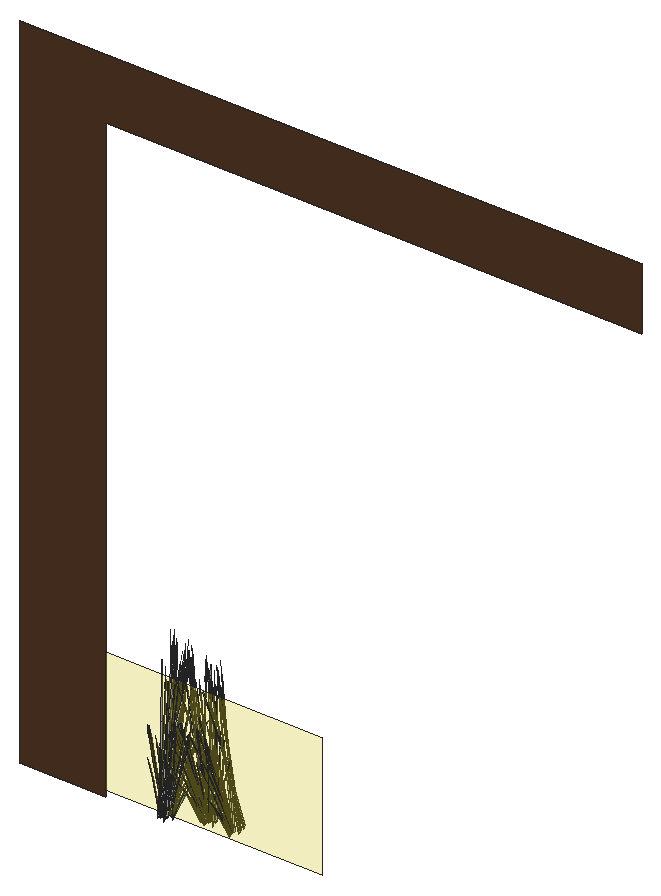
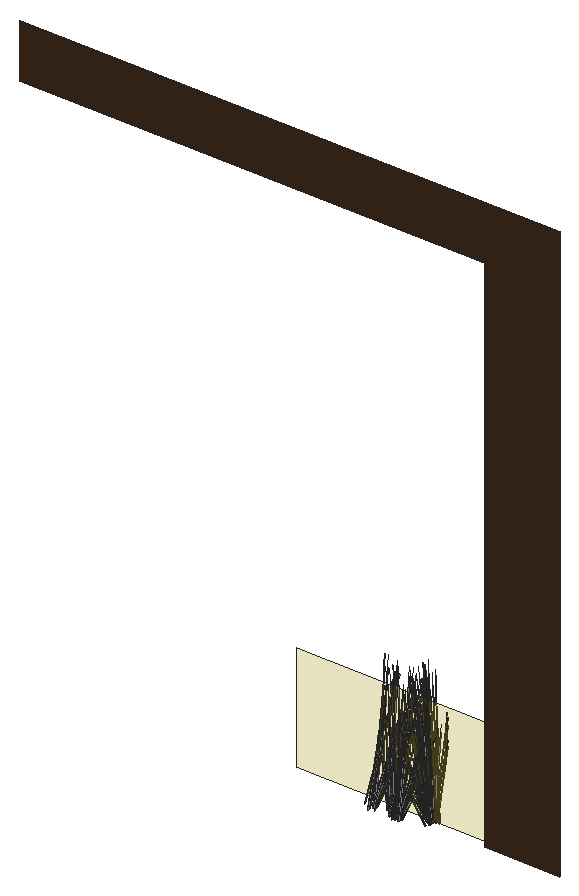
# SketchUp Ruby script. Lengths in inches.
U = 1.inch
M = Sketchup.active_model
def pt(a) = Geom::Point3d.new(a.map { |v| v * U })
def face(e, loops, mat)
  f = e.add_face(loops[0].map { |a| pt(a) })
  loops[1..].each { |l| e.add_face(l.map { |a| pt(a) }).erase! }
  f.material = f.back_material = mat if mat
  f
end
# faces: each face lists its corners as indices into pts; further lists are holes
def faces(e, pts, list, mat = nil) = list.each { |f| face(e, (f[0].is_a?(Array) ? f : [f]).map { |l| l.map { |i| pts[i] } }, mat) }
# xy, xz, yz: faces in a plane at the given z, y or x. An outline is a flat list of corners, or four numbers for a rectangle; further outlines are holes
def ring(l) = l.size == 4 ? [[l[0], l[1]], [l[2], l[1]], [l[2], l[3]], [l[0], l[3]]] : l.each_slice(2).to_a
def flat(e, list, mat, &to3) = list.each { |f| face(e, (f[0].is_a?(Array) ? f : [f]).map { |l| ring(l).map { |u, v| to3.(u, v) } }, mat) }
def xy(e, z, list, mat = nil) = flat(e, list, mat) { |x, y| [x, y, z] }
def xz(e, y, list, mat = nil) = flat(e, list, mat) { |x, z| [x, y, z] }
def yz(e, x, list, mat = nil) = flat(e, list, mat) { |y, z| [x, y, z] }
def lines(e, pts, list) = list.each { |a, b| e.add_line(pt(pts[a]), pt(pts[b])) }
# prism: a flat outline (further loops are holes) pulled along v
def prism(e, loops, v, mat = nil)
  f = face(e, loops, mat); d = Geom::Vector3d.new(v.map { |x| x * U })
  f.pushpull(f.normal.samedirection?(d) ? d.length : -d.length)
end
def box(e, o, s, mat = nil) = prism(e, [[o, [o[0] + s[0], o[1], o[2]], [o[0] + s[0], o[1] + s[1], o[2]], [o[0], o[1] + s[1], o[2]]]], [0, 0, s[2]], mat)
def at(x, y, z, deg = 0) = Geom::Transformation.translation(pt([x, y, z])) * Geom::Transformation.rotation(ORIGIN, Z_AXIS, deg.degrees)
def axes(o, x, y, z) = Geom::Transformation.new([*x, 0, *y, 0, *z, 0, *pt(o).to_a, 1])
def part(name) = M.definitions.add(name)
# library, detail: a bought-in or finely detailed component or shape, given as its bounding box
def library(name, o, s) = part(name).tap { |d| box(d.entities, o, s) }
def detail(e, o, s) = box(e.add_group.entities, o, s)
def put(e, d, t, mat = nil) = e.add_instance(d, t).tap { |i| i.material = mat if mat }
def group(e, t, mat = nil) = e.add_group.tap { |g| g.transformation = t; g.material = mat if mat }.entities
root = M.entities
M.materials.add("Glass_Basic_01").color = [255, 228, 0]
M.materials["Glass_Basic_01"].alpha = 0.25
M.materials.add("LightPink_Translucent").color = [144, 107, 117]
M.materials["LightPink_Translucent"].alpha = 0.75
M.materials.add("Wood_Veneer_15_1K").color = [81, 54, 35]
M.materials.add("[_0053_Ivory_]").color = [200, 200, 200]
c1 = part("blade")
p = [[2.15,0.21,22],[0,0.17,0],[0.09,0.45,0],[2.18,0.31,22],[2.29,0.31,22],[0.38,0.45,0],
  [2.48,0.24,33],[2.49,0.24,33],[2.48,0.22,33]]
faces(c1.entities,p,[[0,1,2,3],[4,5,2,3],[6,3,4,7],[8,0,3,6]])
c2 = part("seeds")
p = [[0.3,-0.1,1.38],[-0.01,-0.03,1.59],[-0.01,-0.03,0.03],[0.14,-0.07,-0.07],[0.29,-0.03,3],[0.15,0.01,3.11]]
faces(c2.entities,p,[[0,1,2,3],[1,0,4,5]],"LightPink_Translucent")
c3 = part("blade with seeds")
put(c3.entities,c1,at(0,0,0))
put(c3.entities,c2,axes([2.4,0.25,30.99],[1.5799,-0.05474,1.17369],[-0.12525,1.92788,0.29478],[-0.07173,-0.02425,1.56792]))
xz(root,98.15,[[410.51,129,494.51,177]],"Glass_Basic_01")
xz(root,98.15,[[377.51,127,410.51,127,410.51,360,617.51,360,617.51,384,377.51,384]],"Wood_Veneer_15_1K")
put(root,c3,axes([433.86,95.57,129.24],[-0.17264,0.12729,1.43002],[-0.51703,-0.22279,-0.30754],[0.09584,-0.27707,0.61141]),"[_0053_Ivory_]")
put(root,c3,axes([434.28,96.52,131.63],[0.0158,-0.58168,-0.71045],[0.66548,0.03907,0.08574],[0.07023,-0.24643,1.00501]),"[_0053_Ivory_]")
put(root,c3,axes([433.53,96.22,130.53],[-0.11309,0.21615,1.71376],[-0.47441,-0.44731,0.13857],[0.21402,-0.27879,0.73262]),"[_0053_Ivory_]")
put(root,c3,axes([434.14,96.32,131.33],[-0.43478,-0.42253,-0.51099],[0.45929,-0.37004,-0.3958],[0.06615,-0.21468,0.97773]),"[_0053_Ivory_]")
put(root,c3,axes([434.55,96.17,131.18],[0.41095,-0.33109,-0.35414],[0.38901,0.37805,0.4572],[0.05919,-0.19208,0.87481]),"[_0053_Ivory_]")
put(root,c3,axes([435.0625,95.97,128.15],[-0.0909,-0.04954,1.76342],[-0.2335,-0.55347,-0.26939],[0.15752,-0.1502,0.30037]),"[_0053_Ivory_]")
put(root,c3,axes([435.0625,97.53,131.63],[0.31725,-0.49618,-0.71045],[0.55593,0.35263,0.08574],[0.18942,-0.17977,1.00501]),"[_0053_Ivory_]")
put(root,c3,axes([435.05,97.3,131.33],[-0.15602,-0.5742,-0.51099],[0.59087,-0.10045,-0.3958],[0.16933,-0.15423,0.97773]),"[_0053_Ivory_]")
put(root,c3,axes([432.15,95.99,128.67],[0.56842,-0.31443,-0.49651],[0.33976,0.56381,0],[0.12946,-0.07161,1.57504]),"[_0053_Ivory_]")
put(root,c3,axes([435.52,97.07,129.24],[-0.21697,-0.01863,1.43002],[-0.22228,-0.49966,-0.30754],[0.26655,-0.14135,0.61141]),"[_0053_Ivory_]")
put(root,c3,axes([432.82,97.28,128.71],[0.40909,-0.47266,-0.62353],[0.50819,0.4286,-0.16365],[0.16393,-0.11791,1.37633]),"[_0053_Ivory_]")
put(root,c3,axes([435.77,96.15,129.42],[-0.2023,0.32011,1.1486],[-0.17388,-0.43009,0.84392],[0.16708,-0.10777,0.25299]),"[_0053_Ivory_]")
put(root,c3,axes([435.48,97.36,131.18],[0.52868,-0.08987,-0.35414],[0.1396,0.51376,0.4572],[0.1515,-0.13799,0.87481]),"[_0053_Ivory_]")
put(root,c3,axes([432.38,97.82,129.32],[-0.07077,-0.71755,-0.29095],[0.73712,-0.04339,-0.50002],[0.1298,-0.09558,1.59708]),"[_0053_Ivory_]")
put(root,c3,axes([432.28,96.23,128.68],[0.56663,0.1556,-0.30978],[-0.14267,0.54795,0.30978],[0.11423,-0.06319,1.38974]),"[_0053_Ivory_]")
put(root,c3,axes([457.25,100.86,130.53],[0.13883,0.2019,1.71376],[-0.64153,0.16998,0.13857],[-0.14499,-0.31697,0.73262]),"[_0053_Ivory_]")
put(root,c3,axes([457.07,100.32,129.24],[-0.03678,0.20572,1.43002],[-0.53767,0.17221,-0.30754],[-0.12568,-0.26589,0.61141]),"[_0053_Ivory_]")
put(root,c3,axes([435.32,98.57,131.33],[0.16454,-0.57202,-0.51099],[0.56413,0.19607,-0.3958],[0.22713,-0.05245,0.97773]),"[_0053_Ivory_]")
put(root,c3,axes([434.43,96.24,129.03],[0.37973,-0.63014,0],[0.6353,0.35142,-0.51607],[0.14469,0.08004,1.63711]),"[_0053_Ivory_]")
put(root,c3,axes([435.92,98.73,128.64],[-0.39118,0.07547,1.41583],[-0.06226,-0.6007,0.08104],[0.27398,-0.09092,0.80566]),"[_0053_Ivory_]")
put(root,c3,axes([436.63,98.2,128.91],[-0.37654,-0.40212,-0.06488],[0.4124,-0.36845,-0.29416],[0.11685,-0.02594,0.97024]),"[_0053_Ivory_]")
put(root,c3,axes([444.76,102.68,130.53],[0.13883,0.2019,1.71376],[-0.64153,0.16998,0.13857],[-0.14499,-0.31697,0.73262]),"[_0053_Ivory_]")
put(root,c3,axes([456.88,99.99,129.42],[0.31682,0.21887,1.1486],[-0.4614,0.13157,0.84392],[-0.09872,-0.16821,0.25299]),"[_0053_Ivory_]")
put(root,c3,axes([434.1,96.57,129.13],[-0.56842,-0.31443,0.49651],[0.33976,-0.56381,0],[0.12946,0.07161,1.57504]),"[_0053_Ivory_]")
put(root,c3,axes([457.65,101.15,131.63],[-0.51789,-0.30395,-0.71045],[0.36805,-0.53263,0.08574],[-0.18764,-0.18149,1.00501]),"[_0053_Ivory_]")
put(root,c3,axes([435.21,98.78,131.63],[0.53369,-0.27773,-0.71045],[0.29743,0.5717,0.08574],[0.25786,-0.06494,1.00501]),"[_0053_Ivory_]")
put(root,c3,axes([457.47,100.75,131.18],[-0.0938,-0.50652,-0.35414],[0.53623,-0.13375,0.4572],[-0.14403,-0.14515,0.87481]),"[_0053_Ivory_]")
put(root,c3,axes([447.26,102.38,129.24],[-0.17264,0.12729,1.43002],[-0.51703,-0.22279,-0.30754],[0.09584,-0.27707,0.61141]),"[_0053_Ivory_]")
put(root,c3,axes([446.47,102.83,131.63],[-0.28988,-0.51132,-0.71045],[0.59671,-0.28496,0.08574],[-0.06778,-0.24706,1.00501]),"[_0053_Ivory_]")
put(root,c3,axes([444.59,102.14,129.24],[-0.03678,0.20572,1.43002],[-0.53767,0.17221,-0.30754],[-0.12568,-0.26589,0.61141]),"[_0053_Ivory_]")
put(root,c3,axes([431.68,97.36,128.25],[-0.59782,0.25177,1.28929],[-0.19028,-0.72239,0.50096],[0.36709,0.01202,1.46642]),"[_0053_Ivory_]")
put(root,c3,axes([433.29,97.55,129.27],[0.11717,-0.56122,0.1448],[0.57245,0.09742,-0.41347],[0.10418,0.05763,1.26744]),"[_0053_Ivory_]")
put(root,c3,axes([445.97,101.69,128.15],[-0.10187,0.02266,1.76342],[-0.56336,-0.25503,-0.26939],[0.00945,-0.21273,0.30037]),"[_0053_Ivory_]")
put(root,c3,axes([456.63,100.65,128.15],[-0.05883,0.08284,1.76342],[-0.59454,0.17861,-0.26939],[-0.14363,-0.16248,0.30037]),"[_0053_Ivory_]")
put(root,c3,axes([436.35,98.34,128.15],[-0.03174,-0.09547,1.76342],[0.22015,-0.55846,-0.26939],[0.22208,-0.00803,0.30037]),"[_0053_Ivory_]")
put(root,c3,axes([456.32,101.49,130.53],[0.2256,0.10835,1.71376],[-0.46687,0.45453,0.13857],[-0.29098,-0.20505,0.73262]),"[_0053_Ivory_]")
put(root,c3,axes([447.68,103.33,131.63],[0.0158,-0.58168,-0.71045],[0.66548,0.03907,0.08574],[0.07023,-0.24643,1.00501]),"[_0053_Ivory_]")
put(root,c3,axes([433.04,97.7,129.37],[-0.36485,-0.52782,0.44739],[0.55265,-0.37168,-0.21531],[0.11807,0.06531,1.43643]),"[_0053_Ivory_]")
put(root,c3,axes([446.53,102.39,131.18],[0.1831,-0.48359,-0.35414],[0.53419,0.14105,0.4572],[-0.04898,-0.1947,0.87481]),"[_0053_Ivory_]")
put(root,c3,axes([446.93,103.03,130.53],[-0.11309,0.21615,1.71376],[-0.47441,-0.44731,0.13857],[0.21402,-0.27879,0.73262]),"[_0053_Ivory_]")
put(root,c3,axes([457.41,101.17,131.33],[-0.59932,0.14948,-0.51099],[-0.10484,-0.56611,-0.3958],[-0.16097,-0.16223,0.97773]),"[_0053_Ivory_]")
put(root,c3,axes([433.23,97.73,129.32],[0.61322,-0.4175,-0.29095],[0.40778,0.58992,-0.50002],[0.1513,0.05991,1.59708]),"[_0053_Ivory_]")
put(root,c3,axes([435.67,98.83,131.18],[0.50475,0.17543,-0.35414],[-0.14722,0.5118,0.4572],[0.20322,-0.04693,0.87481]),"[_0053_Ivory_]")
put(root,c3,axes([446.26,102.72,131.33],[-0.59704,-0.15764,-0.51099],[0.20464,-0.54049,-0.3958],[-0.05475,-0.21761,0.97773]),"[_0053_Ivory_]")
put(root,c3,axes([446.625,101.37,129.42],[0.07791,0.3667,1.1486],[-0.43222,-0.2031,0.84392],[0.04651,-0.18776,0.25299]),"[_0053_Ivory_]")
put(root,c3,axes([434.77,96.62,128.67],[0.56842,0.31443,-0.49651],[-0.33976,0.56381,0],[0.12946,0.07161,1.57504]),"[_0053_Ivory_]")
put(root,c3,axes([433.7,98.42,128.86],[0.67951,0,0],[0,0.65103,0],[0,0,1.78407]),"[_0053_Ivory_]")
put(root,c3,axes([447.55,103.13,131.33],[-0.43478,-0.42253,-0.51099],[0.45929,-0.37004,-0.3958],[0.06615,-0.21468,0.97773]),"[_0053_Ivory_]")
put(root,c3,axes([434.29,98.2,130.53],[-0.25192,0.01424,1.71376],[0.16712,-0.61729,0.13857],[0.35901,0.03818,0.73262]),"[_0053_Ivory_]")
put(root,c3,axes([434.62,96.86,128.68],[0.14267,0.54795,-0.30978],[-0.56663,0.1556,0.30978],[0.11423,0.06319,1.38974]),"[_0053_Ivory_]")
put(root,c3,axes([433.48,98.08,129.03],[-0.76764,-0.13249,0.49198],[0.15622,-0.74829,0.19306],[0.11218,0.07226,1.70813]),"[_0053_Ivory_]")
put(root,c3,axes([447.95,102.98,131.18],[0.41095,-0.33109,-0.35414],[0.38901,0.37805,0.4572],[0.05919,-0.19208,0.87481]),"[_0053_Ivory_]")
put(root,c3,axes([444.4,101.8125,129.42],[0.31682,0.21887,1.1486],[-0.4614,0.13157,0.84392],[-0.09872,-0.16821,0.25299]),"[_0053_Ivory_]")
put(root,c3,axes([445.17,102.97,131.63],[-0.51789,-0.30395,-0.71045],[0.36805,-0.53263,0.08574],[-0.18764,-0.18149,1.00501]),"[_0053_Ivory_]")
put(root,c3,axes([444.99,102.57,131.18],[-0.0938,-0.50652,-0.35414],[0.53623,-0.13375,0.4572],[-0.14403,-0.14515,0.87481]),"[_0053_Ivory_]")
put(root,c3,axes([458.89,104.59,129.98],[0.52485,0.25358,1.51261],[-0.51417,0.54629,0.59816],[-0.23031,-0.32378,1.26806]),"[_0053_Ivory_]")
put(root,c3,axes([433.6,99.86,128.84],[0.63764,-0.21337,-0.19198],[0.22406,0.61462,0.00008],[0.07038,-0.02358,1.73897]),"[_0053_Ivory_]")
put(root,c3,axes([433.95,97.83,128.71],[0.63179,0.1031,-0.62353],[-0.13332,0.63596,-0.16365],[0.18854,0.07706,1.37633]),"[_0053_Ivory_]")
put(root,c3,axes([436.74,98.9375,129.42],[-0.37526,0.10382,1.1486],[0.17664,-0.42906,0.84392],[0.19907,0.02936,0.25299]),"[_0053_Ivory_]")
put(root,c3,axes([444.15,102.47,128.15],[-0.05883,0.08284,1.76342],[-0.59454,0.17861,-0.26939],[-0.14363,-0.16248,0.30037]),"[_0053_Ivory_]")
put(root,c3,axes([445.13,104.75,128.75],[-0.24943,-0.64486,-0.69835],[0.71849,-0.23224,-0.18329],[-0.02757,-0.21836,1.54149]),"[_0053_Ivory_]")
put(root,c3,axes([433.67,98.22,129.37],[0.29468,-0.56664,0.44739],[0.61229,0.27271,-0.21531],[0,0.13062,1.43643]),"[_0053_Ivory_]")
put(root,c3,axes([443.83,103.31,130.53],[0.2256,0.10835,1.71376],[-0.46687,0.45453,0.13857],[-0.29098,-0.20505,0.73262]),"[_0053_Ivory_]")
put(root,c3,axes([448.47,102.78,128.15],[-0.0909,-0.04954,1.76342],[-0.2335,-0.55347,-0.26939],[0.15752,-0.1502,0.30037]),"[_0053_Ivory_]")
put(root,c3,axes([456.23,101.64,131.18],[-0.34557,-0.39372,-0.35414],[0.39459,-0.37271,0.4572],[-0.20048,-0.05671,0.87481]),"[_0053_Ivory_]")
put(root,c3,axes([433.62,98.03,128.86],[0.36485,0.52782,-0.44739],[-0.55265,0.37168,0.21531],[0.11807,0.06531,1.43643]),"[_0053_Ivory_]")
put(root,c3,axes([436.08,100.26,130.58],[-0.11624,-0.52862,-0.03492],[0.54943,-0.12153,-0.15832],[0.11473,0.03351,0.52218]),"[_0053_Ivory_]")
put(root,c3,axes([444.92,102.99,131.33],[-0.59932,0.14948,-0.51099],[-0.10484,-0.56611,-0.3958],[-0.16097,-0.16223,0.97773]),"[_0053_Ivory_]")
put(root,c3,axes([456.26,100.97,128.78],[-0.1752,0.51349,-0.03893],[-0.53924,-0.15795,-0.17649],[-0.08187,-0.08399,0.58215]),"[_0053_Ivory_]")
put(root,c3,axes([435.22,98.54,129.13],[0,-0.62885,0.49651],[0.67951,0,0],[0,0.14322,1.57504]),"[_0053_Ivory_]")
put(root,c3,axes([455.97,103.32,129.03],[-0.75945,0,0],[0,-0.70283,-0.51607],[0,-0.16007,1.63711]),"[_0053_Ivory_]")
put(root,c3,axes([433.93,98.35,129.27],[0.56587,-0.18339,0.1448],[0.19817,0.52368,-0.41347],[0,0.11525,1.26744]),"[_0053_Ivory_]")
put(root,c3,axes([456.1,102.06,129.24],[0.11858,0.17508,1.43002],[-0.27325,0.4759,-0.30754],[-0.28057,-0.11375,0.61141]),"[_0053_Ivory_]")
put(root,c3,axes([448.46,104.34,131.63],[0.31725,-0.49618,-0.71045],[0.55593,0.35263,0.08574],[0.18942,-0.17977,1.00501]),"[_0053_Ivory_]")
put(root,c3,axes([445.03,102.89,129.03],[-0.37973,-0.63014,0],[0.6353,-0.35142,-0.51607],[0.14469,-0.08004,1.63711]),"[_0053_Ivory_]")
put(root,c3,axes([448.45,104.11,131.33],[-0.15602,-0.5742,-0.51099],[0.59087,-0.10045,-0.3958],[0.16933,-0.15423,0.97773]),"[_0053_Ivory_]")
put(root,c3,axes([456.59,101.9,131.63],[-0.60713,-0.01514,-0.71045],[0.04078,-0.63759,0.08574],[-0.25721,-0.06729,1.00501]),"[_0053_Ivory_]")
put(root,c3,axes([445.87,102.13,128.78],[-0.4197,0.36076,-0.03893],[-0.38456,-0.39511,-0.17649],[-0.02707,-0.11196,0.58215]),"[_0053_Ivory_]")
put(root,c3,axes([436.03,99.625,129.24],[-0.14627,-0.15466,1.43002],[0.19032,-0.51164,-0.30754],[0.29594,0.06931,0.61141]),"[_0053_Ivory_]")
put(root,c3,axes([433.42,100.1875,128.86],[0.61229,0.28233,0],[-0.29468,0.58663,0],[0,0,1.74954]),"[_0053_Ivory_]")
put(root,c3,axes([446.41,106.41,129.98],[0.52485,0.25358,1.51261],[-0.51417,0.54629,0.59816],[-0.23031,-0.32378,1.26806]),"[_0053_Ivory_]")
put(root,c3,axes([456.5625,103.13,128.98],[-0.56493,0.5287,0.30756],[-0.56528,-0.52313,-0.36492],[-0.01973,-0.15014,1.64885]),"[_0053_Ivory_]")
put(root,c3,axes([443.66,104.66,128.67],[0,-0.62885,-0.49651],[0.67951,0,0],[0,-0.14322,1.57504]),"[_0053_Ivory_]")
put(root,c3,axes([445.55,102.8,128.67],[0.56842,-0.31443,-0.49651],[0.33976,0.56381,0],[0.12946,-0.07161,1.57504]),"[_0053_Ivory_]")
put(root,c3,axes([448.92,103.88,129.24],[-0.21697,-0.01863,1.43002],[-0.22228,-0.49966,-0.30754],[0.26655,-0.14135,0.61141]),"[_0053_Ivory_]")
put(root,c3,axes([434.69,99.9375,131.63],[0.60713,0.01514,-0.71045],[-0.04078,0.63759,0.08574],[0.25721,0.06729,1.00501]),"[_0053_Ivory_]")
put(root,c3,axes([446.22,104.09,128.71],[0.40909,-0.47266,-0.62353],[0.50819,0.4286,-0.16365],[0.16393,-0.11791,1.37633]),"[_0053_Ivory_]")
put(root,c3,axes([449.17,102.96,129.42],[-0.2023,0.32011,1.1486],[-0.17388,-0.43009,0.84392],[0.16708,-0.10777,0.25299]),"[_0053_Ivory_]")
put(root,c3,axes([456.39,102.03,131.33],[-0.44101,0.41656,-0.51099],[-0.38623,-0.44004,-0.3958],[-0.22407,-0.06338,0.97773]),"[_0053_Ivory_]")
put(root,c3,axes([455.4,102.59,129.42],[0.38775,-0.045,1.1486],[-0.24596,0.39648,0.84392],[-0.19161,-0.05948,0.25299]),"[_0053_Ivory_]")
put(root,c3,axes([448.88,104.17,131.18],[0.52868,-0.08987,-0.35414],[0.1396,0.51376,0.4572],[0.1515,-0.13799,0.87481]),"[_0053_Ivory_]")
put(root,c3,axes([435.68,98.64,129.03],[0.75945,0,0],[0,0.70283,-0.51607],[0,0.16007,1.63711]),"[_0053_Ivory_]")
put(root,c3,axes([433.74,98.39,129.32],[0.68399,0.30005,-0.29095],[-0.32934,0.63331,-0.50002],[0.0215,0.15549,1.59708]),"[_0053_Ivory_]")
put(root,c3,axes([445.51,104.91,128.86],[0.29468,-0.56664,-0.44739],[0.61229,0.27271,0.21531],[0,-0.13062,1.43643]),"[_0053_Ivory_]")
put(root,c3,axes([443.75,103.46,131.18],[-0.34557,-0.39372,-0.35414],[0.39459,-0.37271,0.4572],[-0.20048,-0.05671,0.87481]),"[_0053_Ivory_]")
put(root,c3,axes([445.78,104.63,129.32],[-0.07077,-0.71755,-0.29095],[0.73712,-0.04339,-0.50002],[0.1298,-0.09558,1.59708]),"[_0053_Ivory_]")
put(root,c3,axes([435.06,100.2,131.18],[0.34557,0.39372,-0.35414],[-0.39459,0.37271,0.4572],[0.20048,0.05671,0.87481]),"[_0053_Ivory_]")
put(root,c3,axes([435.22,99.11,128.68],[-0.42396,0.39235,-0.30978],[-0.42396,-0.39235,0.30978],[0,0.12637,1.38974]),"[_0053_Ivory_]")
put(root,c3,axes([455.84,102.48,130.53],[0.25192,-0.01424,1.71376],[-0.16712,0.61729,0.13857],[-0.35901,-0.03818,0.73262]),"[_0053_Ivory_]")
put(root,c3,axes([443.95,104.67,128.68],[0.42396,-0.39235,-0.30978],[0.42396,0.39235,0.30978],[0,-0.12637,1.38974]),"[_0053_Ivory_]")
put(root,c3,axes([443.78,102.79,128.78],[-0.1752,0.51349,-0.03893],[-0.53924,-0.15795,-0.17649],[-0.08187,-0.08399,0.58215]),"[_0053_Ivory_]")
put(root,c3,axes([445.4375,105.38,129.32],[-0.68399,-0.30005,-0.29095],[0.32934,-0.63331,-0.50002],[-0.0215,-0.15549,1.59708]),"[_0053_Ivory_]")
put(root,c3,axes([443.49,105.13,129.03],[-0.75945,0,0],[0,-0.70283,-0.51607],[0,-0.16007,1.63711]),"[_0053_Ivory_]")
put(root,c3,axes([443.62,103.88,129.24],[0.11858,0.17508,1.43002],[-0.27325,0.4759,-0.30754],[-0.28057,-0.11375,0.61141]),"[_0053_Ivory_]")
put(root,c3,axes([445.68,103.04,128.68],[0.56663,0.1556,-0.30978],[-0.14267,0.54795,0.30978],[0.11423,-0.06319,1.38974]),"[_0053_Ivory_]")
put(root,c3,axes([444.11,103.72,131.63],[-0.60713,-0.01514,-0.71045],[0.04078,-0.63759,0.08574],[-0.25721,-0.06729,1.00501]),"[_0053_Ivory_]")
put(root,c3,axes([457.71,104.13,128.71],[-0.63179,-0.1031,-0.62353],[0.13332,-0.63596,-0.16365],[-0.18854,-0.07706,1.37633]),"[_0053_Ivory_]")
put(root,c3,axes([435.51,99.12,128.67],[0,0.62885,-0.49651],[-0.67951,0,0],[0,0.14322,1.57504]),"[_0053_Ivory_]")
put(root,c3,axes([433.8125,99.19,130.53],[-0.2256,-0.10835,1.71376],[0.46687,-0.45453,0.13857],[0.29098,0.20505,0.73262]),"[_0053_Ivory_]")
put(root,c3,axes([444.08,104.95,128.98],[-0.56493,0.5287,0.30756],[-0.56528,-0.52313,-0.36492],[-0.01973,-0.15014,1.64885]),"[_0053_Ivory_]")
put(root,c3,axes([434.65,100.42,129.42],[-0.34197,-0.18082,1.1486],[0.44156,-0.18372,0.84392],[0.1191,0.15563,0.25299]),"[_0053_Ivory_]")
put(root,c3,axes([455.68,103.23,128.15],[0.0154,0.09911,1.76342],[-0.31051,0.51756,-0.26939],[-0.22056,-0.02609,0.30037]),"[_0053_Ivory_]")
put(root,c3,axes([445.875,105.2,129.09],[0.68433,0.30479,0.24065],[-0.32934,0.63331,0.50002],[0,-0.14599,1.60543]),"[_0053_Ivory_]")
put(root,c3,axes([457.04,105.1,128.68],[-0.14267,-0.54795,-0.30978],[0.56663,-0.1556,0.30978],[-0.11423,-0.06319,1.38974]),"[_0053_Ivory_]")
put(root,c3,axes([445.61,106.05,129.09],[0.16098,-0.74515,-0.23429],[0.76326,0.12989,0.51271],[-0.13337,-0.1029,1.5644]),"[_0053_Ivory_]")
put(root,c3,axes([443.91,103.85,131.33],[-0.44101,0.41656,-0.51099],[-0.38623,-0.44004,-0.3958],[-0.22407,-0.06338,0.97773]),"[_0053_Ivory_]")
put(root,c3,axes([442.92,104.4,129.42],[0.38775,-0.045,1.1486],[-0.24596,0.39648,0.84392],[-0.19161,-0.05948,0.25299]),"[_0053_Ivory_]")
put(root,c3,axes([434.75,101.1,128.15],[0.04425,-0.09079,1.76342],[0.55709,-0.26738,-0.26939],[0.16889,0.13839,0.30037]),"[_0053_Ivory_]")
put(root,c3,axes([434.01,99.03,128.75],[0.2227,0.57576,-0.69212],[-0.64151,0.20736,-0.18165],[0.02462,0.19497,1.52773]),"[_0053_Ivory_]")
put(root,c3,axes([456.88,105.34,128.67],[-0.56842,-0.31443,-0.49651],[0.33976,-0.56381,0],[-0.12946,-0.07161,1.57504]),"[_0053_Ivory_]")
put(root,c3,axes([455.62,103.01,131.18],[-0.50475,-0.17543,-0.35414],[0.14722,-0.5118,0.4572],[-0.20322,0.04693,0.87481]),"[_0053_Ivory_]")
put(root,c3,axes([445.66,104.77,129.37],[-0.65953,0.03882,0.44739],[-0.05964,-0.64439,-0.21531],[0.11807,-0.06531,1.43643]),"[_0053_Ivory_]")
put(root,c3,axes([433.88,100.67,131.33],[0.59932,-0.14948,-0.51099],[0.10484,0.56611,-0.3958],[0.16097,0.16223,0.97773]),"[_0053_Ivory_]")
